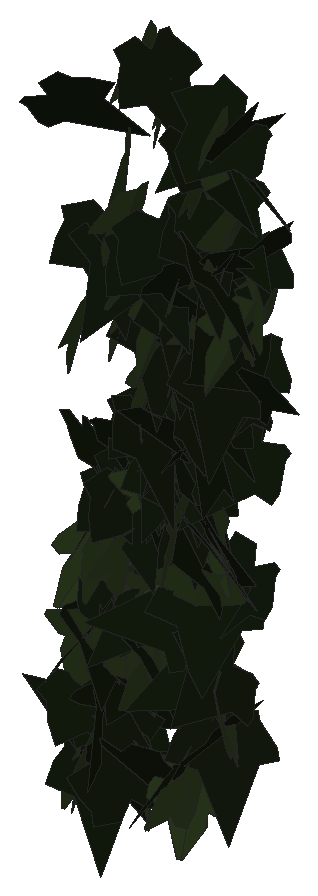
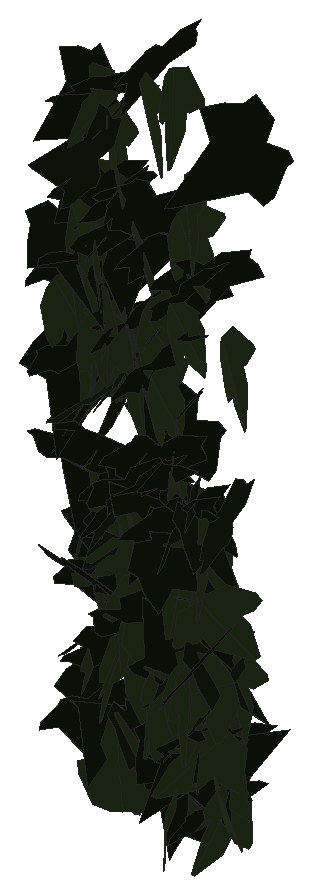
# SketchUp Ruby script. Lengths in inches.
U = 1.inch
M = Sketchup.active_model
def pt(a) = Geom::Point3d.new(a.map { |v| v * U })
def face(e, loops, mat)
  f = e.add_face(loops[0].map { |a| pt(a) })
  loops[1..].each { |l| e.add_face(l.map { |a| pt(a) }).erase! }
  f.material = f.back_material = mat if mat
  f
end
# faces: each face lists its corners as indices into pts; further lists are holes
def faces(e, pts, list, mat = nil) = list.each { |f| face(e, (f[0].is_a?(Array) ? f : [f]).map { |l| l.map { |i| pts[i] } }, mat) }
# xy, xz, yz: faces in a plane at the given z, y or x. An outline is a flat list of corners, or four numbers for a rectangle; further outlines are holes
def ring(l) = l.size == 4 ? [[l[0], l[1]], [l[2], l[1]], [l[2], l[3]], [l[0], l[3]]] : l.each_slice(2).to_a
def flat(e, list, mat, &to3) = list.each { |f| face(e, (f[0].is_a?(Array) ? f : [f]).map { |l| ring(l).map { |u, v| to3.(u, v) } }, mat) }
def xy(e, z, list, mat = nil) = flat(e, list, mat) { |x, y| [x, y, z] }
def xz(e, y, list, mat = nil) = flat(e, list, mat) { |x, z| [x, y, z] }
def yz(e, x, list, mat = nil) = flat(e, list, mat) { |y, z| [x, y, z] }
def lines(e, pts, list) = list.each { |a, b| e.add_line(pt(pts[a]), pt(pts[b])) }
# prism: a flat outline (further loops are holes) pulled along v
def prism(e, loops, v, mat = nil)
  f = face(e, loops, mat); d = Geom::Vector3d.new(v.map { |x| x * U })
  f.pushpull(f.normal.samedirection?(d) ? d.length : -d.length)
end
def box(e, o, s, mat = nil) = prism(e, [[o, [o[0] + s[0], o[1], o[2]], [o[0] + s[0], o[1] + s[1], o[2]], [o[0], o[1] + s[1], o[2]]]], [0, 0, s[2]], mat)
def at(x, y, z, deg = 0) = Geom::Transformation.translation(pt([x, y, z])) * Geom::Transformation.rotation(ORIGIN, Z_AXIS, deg.degrees)
def axes(o, x, y, z) = Geom::Transformation.new([*x, 0, *y, 0, *z, 0, *pt(o).to_a, 1])
def part(name) = M.definitions.add(name)
# library, detail: a bought-in or finely detailed component or shape, given as its bounding box
def library(name, o, s) = part(name).tap { |d| box(d.entities, o, s) }
def detail(e, o, s) = box(e.add_group.entities, o, s)
def put(e, d, t, mat = nil) = e.add_instance(d, t).tap { |i| i.material = mat if mat }
def group(e, t, mat = nil) = e.add_group.tap { |g| g.transformation = t; g.material = mat if mat }.entities
root = M.entities
M.materials.add("efeu1").color = [18, 25, 13]
M.materials.add("efeu2").color = [43, 57, 29]
c1 = part("ivyleaf_9")
p = [[1.54,2.16,1.25],[1.36,2.04,1.19],[-0.21,0.99,0.68],[-0.71,1.11,0.82],[-0.85,0.86,0.67],[-0.8,0.17,0.21],
  [-0.9,-0.01,0.1],[-0.67,-0.16,-0.02],[-0.08,-0.08,-0.05],[-0.03,-0.6,-0.4],[0.65,-0.88,-0.66],[0.83,-0.6,-0.49],
  [1.29,-0.42,-0.43],[1.8125,-0.07,-0.26],[1.21,0.44,0.15]]
faces(c1.entities,p,[[0,1,2,3,4,5,6,7,8,9,10,11,12,13,14]],"efeu1")
c2 = part("ivyleaf_10")
p = [[0,0.5,-0.03],[-0.0625,2.02,-0.43],[-0.19,2.01,-0.46],[-0.54,1.05,-0.29],[-0.52,0.625,-0.18],[-0.83,0.76,-0.28],
  [-1.16,0.64,-0.33],[-1.15,0.33,-0.24],[-0.77,-0.39,0.02],[-0.3,-0.51,0.16],[0.04,-0.48,0.23],[-0.02,2.01,-0.4375],
  [-0.06,2.01,-0.43],[0.04,-0.49,0.23],[0.67,-0.49,0.14],[1.38,0.36,-0.2],[1.375,0.51,-0.24],[0.81,0.65,-0.19],
  [0.62,0.59,-0.15],[0.6,1.09,-0.28],[0.5,1.23,-0.31]]
faces(c2.entities,p,[[0,1,2,3,4,5,6,7,8,9,10],[11,12,0,13,14,15,16,17,18,19,20]],"efeu2")
put(root,c1,axes([28.78,222.86,230.98],[0.07873,-0.44255,-0.21898],[0.00515,0.22247,-0.44775],[0.49374,0.06825,0.03959]))
put(root,c1,axes([29.07,222.77,231.41],[-0.05379,-0.29123,-0.40286],[0.16372,0.37222,-0.29094],[0.46936,-0.16321,0.05531]))
put(root,c2,axes([29.17,222.91,230.75],[0.33627,-0.37002,0.00236],[-0.0039,-0.00673,-0.49994],[0.37001,0.33621,-0.00741]))
put(root,c1,axes([27.93,223.15,224.1],[0.02132,-0.05927,-0.49602],[0.4223,-0.26307,0.04959],[-0.26685,-0.42105,0.03884]))
put(root,c1,axes([29.65,222.69,231.01],[0.13855,0.45207,-0.16261],[-0.0563,-0.15279,-0.47274],[-0.47711,0.1493,0.00857]))
put(root,c1,axes([29.35,223.15,225.72],[-0.28865,-0.06397,0.40322],[-0.34539,-0.22503,-0.28296],[0.21768,-0.44189,0.08572]))
put(root,c1,axes([28.53,222.8,223.08],[-0.28005,-0.3362,0.24195],[0.18315,0.16146,0.43633],[-0.37152,0.33301,0.03272]))
put(root,c1,axes([28.86,222.87,233.7],[0.14229,-0.432,-0.20767],[-0.04722,0.20294,-0.45452],[0.47699,0.14896,0.01695]))
put(root,c1,axes([29.35,223.18,226.59],[0.3245,-0.29691,-0.23779],[0.2006,-0.132,0.43856],[-0.32321,-0.38003,0.03345]))
put(root,c1,axes([27.68,223.18,224.86],[0.06629,-0.3733,0.32596],[0.1218,-0.30651,-0.37579],[0.48038,0.12923,0.0503]))
put(root,c1,axes([29.72,223.14,229.35],[-0.01939,-0.49319,0.07991],[-0.00907,-0.07961,-0.49354],[0.49954,-0.02059,-0.00586]))
put(root,c1,axes([29.48,222.82,232.72],[0.30965,-0.35895,-0.15897],[-0.03349,0.17758,-0.4662],[0.39115,0.29937,0.08594]))
put(root,c1,axes([28.6,223.02,228.36],[0.17735,-0.46748,-0.00377],[-0.00037,0.0039,-0.49998],[0.46749,0.17735,0.00104]))
put(root,c1,axes([28.24,223.25,230.54],[-0.19283,-0.42351,0.18291],[-0.03908,-0.18254,-0.46385],[0.45966,-0.19318,0.03729]))
put(root,c2,axes([29.42,222.77,223.54],[-0.09641,-0.44375,-0.20926],[0.06633,0.19951,-0.45365],[0.48611,-0.11523,0.0204]))
put(root,c1,axes([29.89,223.27,232.92],[-0.3433,-0.29853,0.20743],[-0.05942,-0.23539,-0.43711],[0.35863,-0.32476,0.12614]))
put(root,c1,axes([29.59,223.01,231.04],[0.29687,-0.39726,0.06367],[0.03912,-0.05025,-0.49593],[0.40042,0.29943,0.00124]))
put(root,c2,axes([27.86,222.88,225.05],[-0.44487,-0.06367,0.21918],[-0.21322,-0.05536,-0.44886],[0.08142,-0.49283,0.0221]))
put(root,c2,axes([27.68,222.96,229.68],[0.18815,-0.46325,-0.00104],[0.00245,0.00211,-0.49999],[0.46324,0.18814,0.00306]))
put(root,c1,axes([29.72,223.3125,225.07],[-0.20436,-0.33151,0.31359],[-0.0198,-0.33683,-0.36899],[0.4559,-0.16323,0.12454]))
put(root,c1,axes([27.43,222.64,232.71],[0.41906,0.20429,0.18069],[0.17036,0.06261,-0.46589],[-0.21298,0.45204,-0.01713]))
put(root,c2,axes([28.32,223.05,231.31],[0.04896,-0.48803,0.09712],[0.00538,-0.09707,-0.49046],[0.49757,0.04907,-0.00425]))
put(root,c1,axes([29.5,223.1,231.4],[0.06125,-0.49339,-0.05307],[-0.01234,0.05194,-0.49714],[0.49608,0.06221,-0.00581]))
put(root,c2,axes([28.41,222.94,226.58],[-0.01135,-0.49744,-0.04922],[-0.00431,0.04932,-0.49754],[0.49985,-0.01087,-0.00541]))
put(root,c1,axes([28.47,222.76,223.64],[0.37111,0.25398,-0.21858],[-0.18712,-0.11349,-0.44956],[-0.27797,0.41547,0.01081]))
put(root,c1,axes([27.8125,223.15,223.15],[-0.02339,-0.49919,-0.0162],[0.00192,0.01612,-0.49974],[0.49945,-0.02344,0.00116]))
put(root,c2,axes([29.36,223.19,225.88],[-0.10244,0.08723,0.48156],[-0.29991,-0.39997,0.00865],[0.38673,-0.28708,0.13427]))
put(root,c2,axes([27.71,223.08,223.48],[0.25225,-0.42079,0.09646],[0.04551,-0.08518,-0.49059],[0.4293,0.25628,-0.00467]))
put(root,c2,axes([28.09,222.72,226.51],[0.08804,-0.36127,-0.33426],[0.10466,0.34554,-0.3459],[0.48093,-0.00906,0.13647]))
put(root,c2,axes([29.57,222.94,232.32],[0.1821,-0.45518,-0.09821],[-0.02127,0.09722,-0.49],[0.46517,0.18264,0.01605]))
put(root,c1,axes([29.28,223.01,223.91],[-0.34227,0.31473,-0.18384],[0.1218,-0.13893,-0.46461],[-0.34354,-0.36282,0.01843]))
put(root,c1,axes([28,223.07,230.92],[-0.11498,-0.43754,-0.21294],[0.0696,0.20176,-0.45216],[0.4816,-0.13362,0.01451]))
put(root,c2,axes([29.98,223.24,230.17],[-0.04896,-0.40758,0.28545],[0.03175,-0.2888,-0.40692],[0.49658,-0.02172,0.05416]))
put(root,c2,axes([28.32,223.17,230.11],[0.13905,-0.44279,0.18601],[0.06226,-0.17539,-0.46407],[0.47622,0.15222,0.00636]))
put(root,c1,axes([28.22,223.1,227.3],[-0.18241,-0.27424,-0.37619],[0.35324,0.18164,-0.30369],[0.30323,-0.37656,0.12747]))
put(root,c1,axes([29.39,223.35,228.15],[0.06655,-0.36432,0.33592],[0.04155,-0.33364,-0.37008],[0.49381,0.07717,-0.01413]))
put(root,c2,axes([29.8,223.21,231.44],[0.11425,-0.44066,0.20679],[0.05927,-0.19823,-0.45518],[0.48315,0.12852,0.00694]))
put(root,c1,axes([28.46,222.76,228.35],[0.44558,0.22314,0.04087],[0.03615,0.0191,-0.49833],[-0.22395,0.44704,0.00089]))
put(root,c2,axes([29.3,223.07,223.41],[0.49944,0.0105,0.02119],[0.02124,-0.0021,-0.49954],[-0.0104,0.49989,-0.00254]))
put(root,c2,axes([28.69,223.27,229.93],[0.05781,-0.4092,0.28144],[0.12554,-0.2621,-0.40687],[0.48052,0.1177,0.07244]))
put(root,c2,axes([29.04,223.23,227.16],[0.23676,-0.37944,0.22354],[0.11731,-0.19029,-0.44725],[0.42448,0.26423,-0.00108]))
put(root,c1,axes([29.82,223.08,229.15],[0.13308,0.32888,0.35231],[-0.36131,-0.17382,0.29873],[0.31897,-0.3341,0.1914]))
put(root,c1,axes([28.35,223.23,225.13],[0.25052,-0.38969,0.1881],[0.10027,-0.15915,-0.46327],[0.42093,0.26984,-0.00159]))
put(root,c2,axes([28.78,223.22,227.29],[-0.32517,-0.2474,0.28819],[-0.15053,-0.26437,-0.3968],[0.34872,-0.34482,0.09744]))
put(root,c2,axes([27.82,223.02,223.63],[-0.47642,0.03499,-0.14765],[0.14433,-0.04573,-0.47653],[-0.04685,-0.49667,0.03347]))
put(root,c1,axes([29.51,223.29,226.7],[0.10515,-0.19624,0.4477],[0.25934,-0.36578,-0.22124],[0.41435,0.27873,0.02486]))
put(root,c2,axes([29.51,223.08,226.3],[-0.40456,-0.24453,0.16289],[-0.14814,-0.06962,-0.47245],[0.25374,-0.43053,-0.01612]))
put(root,c1,axes([28.05,223.19,223.51],[0.00978,0.03027,0.49899],[-0.4999,0.00158,0.00971],[-0.00099,-0.49908,0.03029]))
put(root,c1,axes([28.31,223.05,227.32],[0.08906,-0.40098,-0.28511],[-0.02456,0.28575,-0.40956],[0.49139,0.08696,0.0312]))
put(root,c1,axes([29.59,223.44,225.01],[-0.32914,-0.21157,0.3113],[-0.21052,-0.23932,-0.38524],[0.31201,-0.38466,0.06846]))
put(root,c2,axes([28.53,223.3,229.01],[0.13636,-0.42325,0.22862],[0.09911,-0.20781,-0.44384],[0.47073,0.16636,0.02723]))
put(root,c1,axes([29.5,223.29,226.12],[-0.27684,-0.38831,-0.15025],[0.11484,0.10222,-0.47578],[0.40021,-0.29794,0.03259]))
put(root,c1,axes([27.89,223.27,225.5],[-0.35752,0.22627,-0.26642],[0.1626,-0.2297,-0.41328],[-0.30942,-0.38215,0.09066]))
put(root,c2,axes([29.89,222.95,224.75],[-0.25668,0.39611,0.16497],[-0.11528,0.12151,-0.47111],[-0.41331,-0.27988,0.02895]))
put(root,c1,axes([28.09,223.23,227.375],[-0.33325,0.27682,-0.24962],[0.18318,-0.16999,-0.43307],[-0.32463,-0.3801,0.01189]))
put(root,c1,axes([29,223.41,229.92],[-0.02387,-0.49697,0.04953],[-0.00686,-0.04926,-0.49752],[0.49938,-0.02443,-0.00447]))
put(root,c1,axes([27.6,223.07,224.27],[0.11315,-0.34954,-0.33915],[0.09481,0.35733,-0.33664],[0.47771,0.01187,0.14714]))
put(root,c1,axes([29.22,223.31,226.85],[0.27187,-0.32625,0.26391],[0.19448,-0.18068,-0.42371],[0.37184,0.33304,0.02866]))
put(root,c1,axes([28.69,223.45,225.8],[-0.3882,-0.28308,0.13844],[-0.10484,-0.09114,-0.48032],[0.29717,-0.40195,0.01141]))
put(root,c2,axes([29.87,222.78,232.54],[-0.01686,0.02205,0.49923],[-0.20774,0.45399,-0.02707],[-0.45449,-0.20833,-0.00615]))
put(root,c2,axes([28.2,223.12,231.92],[0.21806,-0.42752,-0.14029],[-0.01023,0.15114,-0.4765],[0.44983,0.21068,0.05717]))
put(root,c1,axes([29.92,222.76,232.64],[0.13098,0.2741,0.39713],[0.14611,0.36966,-0.30332],[-0.45989,0.19551,0.01674]))
put(root,c1,axes([29.48,222.9,228.95],[0.26344,-0.10019,-0.41299],[-0.24385,0.36231,-0.24344],[0.34805,0.32968,0.14203]))
put(root,c1,axes([29.64,223.36,224.16],[-0.11644,-0.46685,-0.13598],[0.03098,0.13242,-0.48115],[0.48526,-0.12048,-0.00191]))
put(root,c2,axes([28.79,223.25,233.13],[0.26066,-0.42473,-0.04073],[-0.0107,0.04121,-0.49818],[0.42655,0.26058,0.01239]))
put(root,c2,axes([28.35,223.21,225.4375],[-0.37598,0.2803,-0.17342],[0.1359,-0.10784,-0.46894],[-0.30029,-0.39975,0.00491]))
put(root,c1,axes([27.88,223.6,224.4],[-0.0573,-0.35433,0.34809],[0.07376,-0.35258,-0.34676],[0.4912,0.01161,0.09268]))
put(root,c2,axes([29.03,223.29,229.69],[0.29104,-0.40646,-0.00895],[-0.00514,0.00733,-0.49992],[0.40653,0.29109,0.00009]))
put(root,c2,axes([28.51,223.45,225.34],[-0.29946,-0.2458,-0.31607],[-0.23382,-0.21306,0.38722],[-0.32504,0.37972,0.01266]))
put(root,c2,axes([28.6,222.92,228.06],[0.05043,-0.12584,-0.48127],[-0.17162,0.44964,-0.13555],[0.46691,0.17886,0.00216]))
put(root,c2,axes([27.68,223.36,226.15],[0.30757,0.28254,-0.27491],[-0.21695,-0.16981,-0.41725],[-0.32914,0.37595,0.01814]))
put(root,c1,axes([28.17,223.29,224.21],[0.10587,0.30466,-0.38207],[-0.1024,-0.36842,-0.32215],[-0.47782,0.14645,-0.01562]))
put(root,c2,axes([29.21,223.09,229.14],[-0.32728,0.18084,0.33194],[-0.32177,0.09715,-0.37017],[-0.19838,-0.45591,0.05279]))
put(root,c2,axes([29.33,223.38,227.02],[0.31465,-0.12743,0.36709],[0.35932,-0.0844,-0.33729],[0.14793,0.47606,0.03846]))
put(root,c1,axes([29.39,223.17,229.03],[0.32293,-0.30102,-0.23474],[-0.16802,0.164,-0.44144],[0.34276,0.36399,0.00477]))
put(root,c1,axes([29.67,222.92,224.15],[0.04898,0.47217,0.15704],[0.00319,0.15749,-0.47454],[-0.49758,0.04749,0.01241]))
put(root,c2,axes([28.39,223.18,233.43],[0.07594,-0.46202,-0.17541],[0.01278,0.17924,-0.46659],[0.49403,0.06638,0.03904]))
put(root,c1,axes([28.15,223.58,227.08],[0.09747,-0.34433,0.3492],[0.13257,-0.32428,-0.35675],[0.47215,0.16213,0.02808]))
put(root,c2,axes([28.85,223.28,225.16],[-0.35226,-0.35318,0.03436],[-0.02692,-0.02168,-0.4988],[0.35382,-0.35327,-0.00374]))
put(root,c2,axes([29.75,223.25,231.13],[-0.01164,-0.48928,-0.10231],[-0.00348,0.10241,-0.48939],[0.49985,-0.01068,-0.00579]))
put(root,c1,axes([28.49,223.52,229.54],[-0.02402,-0.49892,0.02237],[-0.00374,-0.02222,-0.49949],[0.49941,-0.02416,-0.00266]))
put(root,c2,axes([27.6,223.04,223.2],[-0.02304,-0.32642,-0.37804],[0.08956,0.36961,-0.3246],[0.49137,-0.08267,0.04144]))
put(root,c1,axes([29.54,223.22,231.77],[0.0682,-0.35976,-0.34048],[-0.00745,0.3429,-0.36381],[0.49527,0.05469,0.04141]))
put(root,c1,axes([27.34,223.4,227.56],[0.3319,-0.36915,0.05978],[0.03328,-0.05045,-0.49633],[0.37247,0.33344,-0.00892]))
put(root,c1,axes([28.89,223.47,227.72],[-0.15616,-0.44618,-0.16291],[0.06823,0.14864,-0.4725],[0.47006,-0.1698,0.01446]))
put(root,c1,axes([28.65,223.65,227.76],[-0.14937,-0.4572,0.1366],[-0.01085,-0.13984,-0.47992],[0.47704,-0.14634,0.03186]))
put(root,c2,axes([29.61,223.29,230.76],[0.27131,-0.3975,-0.13559],[-0.02659,0.14484,-0.47782],[0.41915,0.26649,0.05745]))
put(root,c2,axes([27.95,223.54,225.06],[-0.01358,-0.45136,0.21468],[0.02951,-0.21511,-0.4504],[0.49894,0.00043,0.03248]))
put(root,c1,axes([28.93,223.34,227.84],[-0.23776,0.40109,-0.18053],[0.07574,-0.16482,-0.46594],[-0.43328,-0.24891,0.01761]))
put(root,c1,axes([28.95,223.59,227.41],[0.00546,-0.49957,0.0199],[0.00032,-0.01989,-0.4996],[0.49997,0.00547,0.0001]))
put(root,c2,axes([28.82,223.37,226.58],[0.43334,0.24919,0.01081],[0.00878,0.00642,-0.49988],[-0.24927,0.43343,0.00119]))
put(root,c2,axes([28.125,223.29,226.7],[-0.18861,-0.43316,-0.16369],[0.06513,0.15018,-0.47245],[0.45846,-0.19954,-0.00023]))
put(root,c2,axes([28.8,223.28,225.97],[-0.20423,-0.4187,-0.1816],[0.0775,0.16425,-0.46585],[0.44976,-0.21843,-0.00219]))
put(root,c2,axes([28.51,223.2,224.77],[-0.02595,-0.40518,-0.29181],[0.03326,0.29015,-0.40584],[0.49822,-0.04047,0.01189]))
put(root,c1,axes([28.15,223.23,225.08],[-0.31499,-0.06685,0.38251],[0.37217,0.08852,0.32195],[-0.11077,0.48754,-0.00601]))
put(root,c2,axes([28.15,223.55,224.59],[-0.05654,-0.47739,0.13748],[-0.0022,-0.13813,-0.48054],[0.49679,-0.05494,0.01352]))
put(root,c2,axes([29.32,223.48,229.76],[-0.0947,-0.48803,0.05342],[-0.01552,-0.05141,-0.49711],[0.4907,-0.09582,-0.00541]))
put(root,c2,axes([29.59,223.31,229.68],[0.19703,-0.40936,-0.20881],[-0.0177,0.22026,-0.44852],[0.4592,0.18414,0.07231]))
put(root,c1,axes([28.96,223.59,227.42],[0.26928,-0.40325,0.12197],[0.05303,-0.11116,-0.48459],[0.41794,0.27392,-0.0171]))
put(root,c2,axes([27.81,223.36,227.125],[0.19642,-0.41759,-0.19245],[0.00162,0.2099,-0.4538],[0.4598,0.17765,0.08381]))
put(root,c2,axes([27.64,223.33,224.16],[-0.22912,-0.27746,-0.34716],[0.33716,0.14593,-0.33916],[0.28952,-0.38951,0.12023]))
put(root,c1,axes([28.74,223.66,229.49],[0.18067,-0.45558,0.09902],[0.03972,-0.09077,-0.49008],[0.46452,0.18496,0.00339]))
put(root,c1,axes([29.68,223.71,229.46],[-0.2094,-0.45375,-0.0162],[0.0069,0.01466,-0.49974],[0.45398,-0.20952,0.00012]))
put(root,c2,axes([29,223.52,223.14],[-0.45059,-0.21159,0.04687],[0.04375,0.0171,0.49779],[-0.21225,0.4527,0.00311]))
put(root,c1,axes([29.36,223.84,228.8],[-0.1284,-0.41802,0.24243],[0.12127,-0.27069,-0.40252],[0.46777,-0.04457,0.1709]))
put(root,c2,axes([27.53,223.44,225.13],[-0.26855,0.05732,-0.41785],[0.414,-0.05878,-0.27414],[-0.08055,-0.49321,-0.01589]))
put(root,c1,axes([29.72,223.72,226.28],[-0.46674,-0.10996,-0.14163],[0.16315,-0.09662,-0.46265],[0.07437,-0.47809,0.12607]))
put(root,c1,axes([28.3,223.72,227.09],[-0.25873,0.16225,-0.3959],[0.17874,-0.37936,-0.27228],[-0.38873,-0.28242,0.13831]))
put(root,c2,axes([29.55,223.4,230],[-0.45453,0.16998,0.12044],[-0.12947,-0.00401,-0.48293],[-0.16321,-0.4702,0.04766]))
put(root,c1,axes([29.98,223.41,231.06],[-0.10602,0.45738,-0.17194],[0.00596,-0.17472,-0.46844],[-0.48859,-0.10138,0.0316]))
put(root,c2,axes([28.05,223.73,223.125],[0.09155,-0.31847,0.37443],[0.33741,-0.23626,-0.28344],[0.35746,0.30457,0.17165]))
put(root,c1,axes([28.72,223.76,227.86],[-0.26843,-0.42183,0.00193],[-0.00299,-0.00039,-0.49999],[0.42183,-0.26844,-0.00232]))
put(root,c1,axes([27.75,223.37,224.15],[0.03617,-0.30002,-0.39835],[0.03597,0.39992,-0.29794],[0.49739,-0.0071,0.05051]))
put(root,c1,axes([28.43,223.49,228.31],[-0.0514,-0.38151,-0.31907],[0.07603,0.31098,-0.38407],[0.49151,-0.088,0.02604]))
put(root,c2,axes([29.34,223.42,229.66],[-0.48918,0.09439,-0.04233],[0.04343,0.00169,-0.49811],[-0.09389,-0.49101,-0.00985]))
put(root,c1,axes([29.8,223.32,229.24],[0.38972,0.21575,-0.22708],[-0.21247,-0.08426,-0.4447],[-0.23016,0.44312,0.02601]))
put(root,c2,axes([29.16,223.42,225.01],[-0.24962,0.4332,-0.00506],[0.0006,-0.00549,-0.49997],[-0.43323,-0.24961,0.00222]))
put(root,c2,axes([29.78,223.7,230.17],[-0.04216,-0.45014,0.21353],[-0.01053,-0.21344,-0.45203],[0.49811,-0.04261,0.00852]))
put(root,c1,axes([28.16,223.5,227.43],[0.04036,-0.41066,-0.28237],[0.02039,0.28442,-0.41072],[0.49795,0.02164,0.0397]))
put(root,c1,axes([28.74,223.79,225.98],[-0.36937,-0.32751,0.07939],[-0.05968,-0.05235,-0.49366],[0.33166,-0.37416,-0.00042]))
put(root,c1,axes([27.65,223.875,225.42],[-0.03719,-0.41753,0.27255],[0.01642,-0.27418,-0.4178],[0.49834,-0.02213,0.03411]))
put(root,c2,axes([29.87,223.47,230.29],[0.423,-0.22857,-0.13722],[-0.07861,0.13898,-0.47382],[0.25475,0.42242,0.08164]))
put(root,c1,axes([29.82,223.73,228.1],[-0.46734,-0.17512,0.03037],[-0.02689,-0.01479,-0.49906],[0.17569,-0.46809,0.00441]))
put(root,c1,axes([29.35,223.62,232.26],[0.33295,-0.3182,0.19465],[0.16527,-0.10807,-0.45936],[0.33441,0.37023,0.03321]))
put(root,c1,axes([29.66,223.75,230.86],[-0.11507,-0.48548,-0.03269],[-0.00068,0.03375,-0.49886],[0.48658,-0.11476,-0.00843]))
put(root,c2,axes([27.9,223.45,225.01],[0.00244,-0.47681,-0.1505],[0.03554,0.15029,-0.47555],[0.49873,-0.00838,0.03463]))
